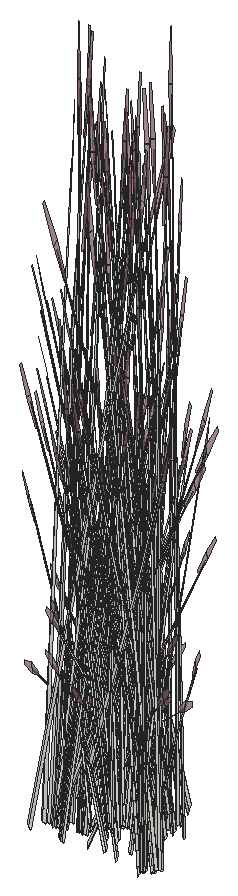
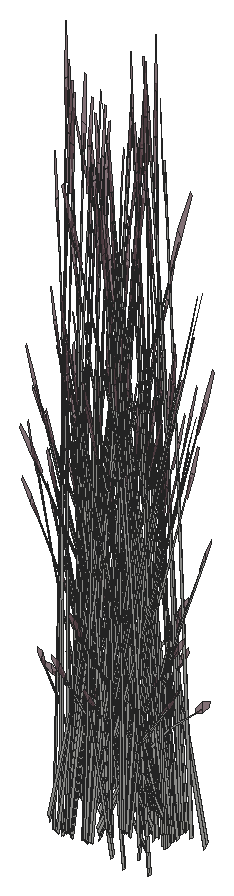
# SketchUp Ruby script. Lengths in inches.
U = 1.inch
M = Sketchup.active_model
def pt(a) = Geom::Point3d.new(a.map { |v| v * U })
def face(e, loops, mat)
  f = e.add_face(loops[0].map { |a| pt(a) })
  loops[1..].each { |l| e.add_face(l.map { |a| pt(a) }).erase! }
  f.material = f.back_material = mat if mat
  f
end
# faces: each face lists its corners as indices into pts; further lists are holes
def faces(e, pts, list, mat = nil) = list.each { |f| face(e, (f[0].is_a?(Array) ? f : [f]).map { |l| l.map { |i| pts[i] } }, mat) }
# xy, xz, yz: faces in a plane at the given z, y or x. An outline is a flat list of corners, or four numbers for a rectangle; further outlines are holes
def ring(l) = l.size == 4 ? [[l[0], l[1]], [l[2], l[1]], [l[2], l[3]], [l[0], l[3]]] : l.each_slice(2).to_a
def flat(e, list, mat, &to3) = list.each { |f| face(e, (f[0].is_a?(Array) ? f : [f]).map { |l| ring(l).map { |u, v| to3.(u, v) } }, mat) }
def xy(e, z, list, mat = nil) = flat(e, list, mat) { |x, y| [x, y, z] }
def xz(e, y, list, mat = nil) = flat(e, list, mat) { |x, z| [x, y, z] }
def yz(e, x, list, mat = nil) = flat(e, list, mat) { |y, z| [x, y, z] }
def lines(e, pts, list) = list.each { |a, b| e.add_line(pt(pts[a]), pt(pts[b])) }
# prism: a flat outline (further loops are holes) pulled along v
def prism(e, loops, v, mat = nil)
  f = face(e, loops, mat); d = Geom::Vector3d.new(v.map { |x| x * U })
  f.pushpull(f.normal.samedirection?(d) ? d.length : -d.length)
end
def box(e, o, s, mat = nil) = prism(e, [[o, [o[0] + s[0], o[1], o[2]], [o[0] + s[0], o[1] + s[1], o[2]], [o[0], o[1] + s[1], o[2]]]], [0, 0, s[2]], mat)
def at(x, y, z, deg = 0) = Geom::Transformation.translation(pt([x, y, z])) * Geom::Transformation.rotation(ORIGIN, Z_AXIS, deg.degrees)
def axes(o, x, y, z) = Geom::Transformation.new([*x, 0, *y, 0, *z, 0, *pt(o).to_a, 1])
def part(name) = M.definitions.add(name)
# library, detail: a bought-in or finely detailed component or shape, given as its bounding box
def library(name, o, s) = part(name).tap { |d| box(d.entities, o, s) }
def detail(e, o, s) = box(e.add_group.entities, o, s)
def put(e, d, t, mat = nil) = e.add_instance(d, t).tap { |i| i.material = mat if mat }
def group(e, t, mat = nil) = e.add_group.tap { |g| g.transformation = t; g.material = mat if mat }.entities
root = M.entities
M.materials.add("LightPink_Translucent").color = [144, 107, 117]
M.materials["LightPink_Translucent"].alpha = 0.75
c1 = part("blade")
p = [[2.15,0.21,22],[0,0.17,0],[0.09,0.45,0],[2.18,0.31,22],[2.29,0.31,22],[0.38,0.45,0],
  [2.48,0.24,33],[2.49,0.24,33],[2.48,0.22,33]]
faces(c1.entities,p,[[0,1,2,3],[4,5,2,3],[6,3,4,7],[8,0,3,6]])
c2 = part("seeds")
p = [[0.3,-0.1,1.38],[-0.01,-0.03,1.59],[-0.01,-0.03,0.03],[0.14,-0.07,-0.07],[0.29,-0.03,3],[0.15,0.01,3.11]]
faces(c2.entities,p,[[0,1,2,3],[1,0,4,5]],"LightPink_Translucent")
c3 = part("blade with seeds")
put(c3.entities,c1,at(0,0,0))
put(c3.entities,c2,axes([2.4,0.25,30.99],[1.5799,-0.05474,1.17369],[-0.12525,1.92788,0.29478],[-0.07173,-0.02425,1.56792]))
put(root,c3,axes([316.8125,31.4,46.4],[0.44368,-0.17257,-0.62776],[0.24726,0.35524,0.07576],[0.21437,-0.04035,0.88802]))
put(root,c3,axes([314.82,30.79,44.09],[-0.41865,0.35461,0.40429],[-0.49737,-0.31303,0.15865],[0.10093,-0.03539,1.40366]))
put(root,c3,axes([321.99,33.24,46],[0.15222,-0.30049,-0.31292],[0.44409,0.08764,0.40398],[-0.04072,-0.12098,0.77298]))
put(root,c3,axes([323.45,30.63,43.9375],[-0.31175,-0.39292,-0.04544],[0.52815,-0.21836,0.456],[-0.13015,0.03741,1.44584]))
put(root,c3,axes([316.75,31.47,46.46],[-0.41962,-0.10901,0.31292],[0.12239,-0.31802,-0.40398],[0.16894,-0.02916,0.77298]))
put(root,c3,axes([323.34,29.68,44.3125],[0.37303,0.23477,0.12794],[-0.31115,0.26487,-0.36534],[-0.08661,0.03581,1.11991]))
put(root,c3,axes([320.4,29.74,46.18],[-0.12522,-0.35963,0.42415],[0.49122,-0.06241,0.34973],[-0.14477,0.08458,0.87768]))
put(root,c3,axes([320.3,29.67,46.18],[-0.34663,-0.16434,0.05682],[0.20181,-0.23402,0.44729],[-0.11113,0.07566,0.68204]))
put(root,c3,axes([321.76,33.44,46.14],[-0.49634,-0.09796,-0.45151],[0.17013,-0.33585,-0.34973],[-0.04551,-0.13522,0.86392]))
put(root,c3,axes([313.875,30.52,43.41],[-0.49699,0.15644,1.13921],[-0.15819,-0.44887,0.44265],[0.30518,0.00747,1.29573]))
put(root,c3,axes([315.21,30.64,44.3125],[0.09741,-0.34873,0.12794],[0.4759,0.06053,-0.36534],[0.08661,0.03581,1.11991]))
put(root,c3,axes([317.76,31.125,43.32],[-0.02639,-0.05932,1.55816],[0.18302,-0.34702,-0.23804],[0.18462,-0.00499,0.26541]))
put(root,c3,axes([320.875,32.4,46.16],[-0.00942,0.04684,1.56736],[-0.46458,0.16998,-0.1481],[-0.13671,-0.08689,0.27737]))
put(root,c3,axes([315.01,30.73,44.4],[-0.30332,-0.32798,0.39531],[0.45944,-0.23096,-0.19025],[0.09816,0.04058,1.26923]))
put(root,c3,axes([323.74,30.4,44.19],[0.47255,-0.19538,0.43871],[0.28245,0.35034,0],[-0.10763,0.0445,1.3917]))
put(root,c3,axes([320.77,33.23,46.5],[0.56246,-0.10044,0.47505],[0.09762,0.39398,0.3917],[-0.13228,-0.11611,0.983]))
put(root,c3,axes([323.3125,30.58,43.79],[-0.47106,-0.09668,-0.27372],[0.11861,-0.34048,0.27372],[-0.09497,0.03926,1.22797]))
put(root,c3,axes([319.91,29.89,44.29],[0.17547,0.03208,1.26356],[0.1131,0.32764,-0.27174],[-0.23835,0.06133,0.54024]))
put(root,c3,axes([315.16,30.75,44.36],[0.50979,-0.25942,-0.25709],[0.339,0.36656,-0.44182],[0.12578,0.03723,1.41118]))
put(root,c3,axes([317.19,31.43,46],[0.41962,0.10901,-0.31292],[-0.12239,0.31802,0.40398],[0.16894,-0.02916,0.77298]))
put(root,c3,axes([322.04,33.31,46.18],[0.49753,0.10215,0.42415],[-0.17013,0.33585,0.34973],[-0.0299,-0.13207,0.87768]))
put(root,c3,axes([322.1875,33.43,46.45],[-0.49409,0.18193,-0.10745],[-0.24281,-0.32289,-0.59638],[-0.06519,-0.13607,0.90619]))
put(root,c3,axes([320.7,29.62,46.46],[0.43951,-0.05584,0.31292],[0.11606,0.31924,-0.40398],[-0.12595,0.08575,0.77298]))
put(root,c3,axes([320.22,32.875,44.44],[0.26338,0.136,1.01491],[-0.38358,0.08175,0.74569],[-0.08207,-0.10452,0.22354]))
put(root,c3,axes([319.01,29.48,46.16],[0.06444,0.01048,1.56736],[0.19934,0.34525,-0.1481],[-0.13191,0.09062,0.27737]))
put(root,c3,axes([322.18,33.28,46.18],[0.37205,-0.1328,0.05682],[0.18211,0.24217,0.44729],[-0.03593,-0.10675,0.68204]))
put(root,c3,axes([320.86,33.6,46.4],[-0.43054,-0.18887,-0.62776],[0.30598,-0.33097,0.07576],[-0.15599,-0.11277,0.88802]))
put(root,c3,axes([316.45,30.06,43.78],[0.47255,0.19538,-0.43871],[-0.28245,0.35034,0],[0.10763,0.0445,1.3917]))
put(root,c3,axes([320.71,33.35,46],[-0.07798,-0.31474,-0.31292],[0.44579,-0.08311,0.40398],[-0.11974,-0.09019,0.77298]))
put(root,c3,axes([315.55,31.17,43.95],[0.56491,0,0],[0,0.40454,0],[0,0,1.5764]))
put(root,c3,axes([319.55,30.57,44.44],[0.21042,-0.1771,1.01491],[0.08303,0.28036,0.74569],[-0.15207,0.0502,0.22354]))
put(root,c3,axes([323.23,29.59,44.36],[0.05884,0.44587,-0.25709],[-0.6128,0.02696,-0.44182],[-0.10791,0.05939,1.41118]))
put(root,c3,axes([320.34,29.81,46],[-0.43951,0.05584,-0.31292],[-0.11606,-0.31924,0.40398],[-0.12595,0.08575,0.77298]))
put(root,c3,axes([316.05,31.04,45.43],[-0.20943,0.00885,1.51428],[0.13893,-0.38357,0.12244],[0.29846,0.02372,0.64734]))
put(root,c3,axes([316.32,30.21,43.79],[0.11861,0.34048,-0.27372],[-0.47106,0.09668,0.27372],[0.09497,0.03926,1.22797]))
put(root,c3,axes([317.13,31.57,46.18],[0.18545,0.26643,0.05682],[-0.33817,0.13041,0.44729],[0.14907,-0.02573,0.68204]))
put(root,c3,axes([320.9,33.32,46.18],[0.22948,-0.24822,0.05682],[0.32679,0.14452,0.44729],[-0.10565,-0.07958,0.68204]))
put(root,c3,axes([320.01,33.28,43.32],[-0.04891,0.05148,1.55816],[-0.49427,0.11098,-0.23804],[-0.1194,-0.10096,0.26541]))
put(root,c3,axes([315.37,30.97,44.1],[-0.63817,-0.08233,0.43472],[0.12987,-0.46497,0.17059],[0.09326,0.0449,1.50931]))
put(root,c3,axes([317.09,31.47,46.18],[-0.14265,0.35629,0.42415],[-0.46898,-0.12183,0.34973],[0.18443,-0.02141,0.87768]))
put(root,c3,axes([319.7,30.53,46.99],[0.44556,0.1043,-0.05733],[-0.13706,0.32103,-0.25992],[-0.07288,0.04874,0.85731]))
put(root,c3,axes([322.86,29.93,43.82],[-0.34009,0.2937,-0.55095],[-0.42248,-0.26632,-0.1446],[-0.13628,0.07327,1.21613]))
put(root,c3,axes([320.83,34.7,43.85],[-0.20736,-0.4007,-0.61707],[0.59731,-0.14431,-0.16195],[-0.02292,-0.13569,1.36206]))
put(root,c3,axes([315.48,32.07,43.93],[0.53009,-0.13258,-0.16963],[0.18627,0.38191,0.00007],[0.05851,-0.01465,1.53656]))
put(root,c3,axes([323.47,30.43,44.06],[0.63212,0.12701,0.27176],[-0.15814,0.45398,-0.32244],[-0.10462,0.05682,1.45692]))
put(root,c3,axes([323.42,30.73,43.78],[-0.47255,0.19538,-0.43871],[-0.28245,-0.35034,0],[-0.10763,0.0445,1.3917]))
put(root,c3,axes([315.54,31.35,43.96],[0.35245,0.2524,0],[-0.35245,0.2524,0],[0,0,1.49564]))
put(root,c3,axes([322.04,33.55,46.46],[-0.15222,0.30049,0.31292],[-0.44409,-0.08764,-0.40398],[-0.04072,-0.12098,0.77298]))
put(root,c3,axes([320.66,33.6,46.14],[-0.49824,0.09289,-0.45151],[-0.08716,-0.35177,-0.34973],[-0.13382,-0.10081,0.86392]))
put(root,c3,axes([315.76,30.81,43.82],[0.52523,0.06406,-0.55095],[-0.11084,0.39517,-0.1446],[0.15674,0.04788,1.21613]))
put(root,c3,axes([318.08,31.5,44.44],[-0.31197,0.06451,1.01491],[0.14684,-0.26661,0.74569],[0.1655,0.01824,0.22354]))
put(root,c3,axes([321,33.29,46.8],[-0.33698,0.3746,-0.12034],[-0.48801,-0.21581,-0.66795],[-0.16964,-0.10584,1.01494]))
put(root,c3,axes([320.47,29.59,46.45],[0.46706,0.21546,-0.10745],[-0.26908,0.31203,-0.59638],[-0.13196,0.10846,0.90619]))
put(root,c3,axes([320.75,33.55,44.1],[-0.31568,-0.39156,0],[0.52815,-0.21836,-0.456],[0.12029,-0.04973,1.44655]))
put(root,c3,axes([315.46,35.08,44.29],[-0.14352,0.07909,1.26356],[-0.42983,-0.13843,-0.27174],[0.07968,-0.17216,0.54024]))
put(root,c3,axes([315.53,31.05,44.4],[0.24498,-0.3521,0.39531],[0.50902,0.16945,-0.19025],[0,0.08116,1.26923]))
put(root,c3,axes([321.1,29.49,45.43],[0.12611,-0.12006,1.51428],[0.31843,0.32408,0.12244],[-0.2184,0.14759,0.64734]))
put(root,c3,axes([317.94,32.625,46.16],[-0.04566,-0.03421,1.56736],[0.09987,-0.36669,-0.1481],[0.17984,-0.02343,0.27737]))
put(root,c3,axes([321.44,33.08,43.88],[-0.34892,0.22417,-0.0344],[-0.3197,-0.24551,-0.15595],[-0.02251,-0.06957,0.51438]))
put(root,c3,axes([320.7,29.85,46.14],[0.12971,0.3568,-0.45151],[-0.49122,0.06241,-0.34973],[-0.14077,0.09583,0.86392]))
put(root,c3,axes([321.29,30.26,46.46],[0.34164,-0.20573,0.31292],[0.3234,0.23491,-0.40398],[-0.04921,0.11936,0.77298]))
put(root,c3,axes([323.85,30.67,44.1],[0.31568,0.39156,0],[-0.52815,0.21836,-0.456],[-0.12029,0.04973,1.44655]))
put(root,c3,axes([315.49,30.93,43.95],[0.30332,0.32798,-0.39531],[-0.45944,0.23096,0.19025],[0.09816,0.04058,1.26923]))
put(root,c3,axes([317.54,32.32,45.47],[-0.09664,-0.32847,-0.03085],[0.45676,-0.07551,-0.13989],[0.09538,0.02082,0.4614]))
put(root,c3,axes([319.71,33.18,46.17],[-0.10864,-0.00276,1.54581],[-0.34587,0.27582,-0.24447],[-0.18454,-0.05636,0.12397]))
put(root,c3,axes([316.35,32.31,46.45],[0.02704,-0.39739,-0.10745],[0.51189,0.01086,-0.59638],[0.19715,0.0276,0.90619]))
put(root,c3,axes([323.58,29.12,44.51],[-0.01379,-0.36791,1.24828],[0.62424,0.09537,0.52853],[-0.14764,0.20132,1.17828]))
put(root,c3,axes([320.98,30.44,46.18],[-0.41493,-0.01821,0.05682],[0.01138,-0.27493,0.44729],[-0.04342,0.10531,0.68204]))
put(root,c3,axes([320.1,30.76,43.32],[0.06773,0.03904,1.55816],[0.11484,0.36171,-0.23804],[-0.15011,0.07713,0.26541]))
put(root,c3,axes([316.82,31.25,44.19],[0,-0.39075,0.43871],[0.56491,0,0],[0,0.089,1.3917]))
put(root,c3,axes([321.12,30.47,46.18],[-0.35954,-0.26661,0.42415],[0.38183,-0.22994,0.34973],[-0.06632,0.12508,0.87768]))
put(root,c3,axes([315.75,31.13,44.3125],[0.47043,-0.11396,0.12794],[0.16474,0.32541,-0.36534],[0,0.07162,1.11991]))
put(root,c3,axes([315.8125,35.67,46.4],[0.01314,-0.36145,-0.62776],[0.55324,0.02428,0.07576],[0.05838,-0.15313,0.88802]))
put(root,c3,axes([321.89,35.73,44.9375],[0.43633,0.15757,1.33654],[-0.42745,0.33945,0.52853],[-0.19146,-0.20119,1.12046]))
put(root,c3,axes([316.28,32.15,46.46],[-0.28729,-0.24465,0.31292],[0.32804,-0.23159,-0.40398],[0.16667,0.03524,0.77298]))
put(root,c3,axes([320.97,33.6,46.46],[0.07798,0.31474,0.31292],[-0.44579,0.08311,-0.40398],[-0.11974,-0.09019,0.77298]))
put(root,c3,axes([319.61,34.64,43.78],[0,-0.39075,-0.43871],[0.56491,0,0],[0,-0.089,1.3917]))
put(root,c3,axes([316.58,35.1,46.17],[-0.00487,-0.07777,1.54581],[-0.41166,-0.22476,-0.24447],[0.06364,-0.13625,0.12397]))
put(root,c3,axes([315.19,35.48,45.43],[-0.09401,0.13431,1.51428],[-0.3944,-0.27795,0.12244],[0.17792,-0.17323,0.64734]))
put(root,c3,axes([316.47,34.82,46.16],[-0.05128,0.02985,1.56736],[-0.5024,-0.1007,-0.1481],[-0.01819,-0.13025,0.27737]))
put(root,c3,axes([319.63,33.81,46.5],[0.41698,-0.28837,0.47505],[0.35962,0.30624,0.3917],[-0.19563,-0.05319,0.983]))
put(root,c3,axes([317.5,31.93,44.29],[-0.1216,-0.0961,1.26356],[0.15822,-0.31792,-0.27174],[0.24603,0.04307,0.54024]))
put(root,c3,axes([315.32,32.27,43.95],[0.50902,0.17543,0],[-0.24498,0.36452,0],[0,0,1.54589]))
put(root,c3,axes([315.7,35.55,46.14],[-0.36145,-0.26255,-0.45151],[0.38183,-0.22994,-0.34973],[0.055,-0.1334,0.86392]))
put(root,c3,axes([316.8,32.07,46.17],[0.10831,-0.00661,1.54581],[0.29709,-0.30358,-0.24447],[0.19266,0.04007,0.12397]))
put(root,c3,axes([321.01,29.79,45.43],[0.09401,-0.13431,1.51428],[0.3944,0.27795,0.12244],[-0.17792,0.17323,0.64734]))
put(root,c3,axes([319.82,33.81,46.18],[0.02542,-0.29714,0.05682],[0.38391,0.00815,0.44729],[-0.14706,-0.03109,0.68204]))
put(root,c3,axes([321.14,34.8,43.95],[0.24498,-0.3521,-0.39531],[0.50902,0.16945,0.19025],[0,-0.08116,1.26923]))
put(root,c3,axes([319.68,33.9,46],[-0.28729,-0.24465,-0.31292],[0.32804,-0.23159,0.40398],[-0.16667,-0.03524,0.77298]))
put(root,c3,axes([319.85,34.65,43.79],[0.35245,-0.2438,-0.27372],[0.35245,0.2438,0.27372],[0,-0.07853,1.22797]))
put(root,c3,axes([322.11,30.87,46.18],[-0.37205,0.1328,0.05682],[-0.18211,-0.24217,0.44729],[0.03593,0.10675,0.68204]))
put(root,c3,axes([321.11,30.55,46],[-0.34164,0.20573,-0.31292],[-0.3234,-0.23491,0.40398],[-0.04921,0.11936,0.77298]))
put(root,c3,axes([319.9375,30.49,46.17],[-0.01255,0.07733,1.54581],[0.35618,0.269,-0.24447],[-0.09325,0.12721,0.12397]))
put(root,c3,axes([316.38,32.12,46.4],[0.50473,0.00941,-0.62776],[-0.0339,0.39618,0.07576],[0.21383,0.04181,0.88802]))
put(root,c3,axes([321.08,30.3125,46.77],[0.55492,0.01936,-0.11927],[-0.01517,0.36657,-0.66198],[-0.03855,0.14118,1.00587]))
put(root,c3,axes([319.71,33.48,43.88],[-0.14565,0.31907,-0.0344],[-0.44829,-0.09815,-0.15595],[-0.06806,-0.05219,0.51438]))
put(root,c3,axes([321.08,35.09,44.36],[-0.56863,-0.18645,-0.25709],[0.2738,-0.39352,-0.44182],[-0.01787,-0.09662,1.41118]))
put(root,c3,axes([322.25,30.84,46.47],[-0.49753,-0.10215,0.47081],[0.17013,-0.33585,0.3882],[0.0299,0.13207,0.97422]))
put(root,c3,axes([316.08,35.68,46.45],[-0.55492,-0.01936,-0.10745],[0.01517,-0.36657,-0.59638],[0.03855,-0.14118,0.90619]))
put(root,c3,axes([316.04,35.45,46],[0.34164,-0.20573,-0.31292],[0.3234,0.23491,0.40398],[0.04921,-0.11936,0.77298]))
put(root,c3,axes([319.47,34.9375,44.1],[-0.63136,0,0],[0,-0.43672,-0.456],[0,-0.09947,1.44655]))
put(root,c3,axes([321.33,31.35,44.44],[-0.01307,-0.23234,1.01491],[0.32652,0.16572,0.74569],[-0.06422,0.11074,0.22354]))
put(root,c3,axes([322.19,30.79,43.32],[0.08172,-0.02126,1.55816],[0.49154,0.11703,-0.23804],[0.01437,0.1319,0.26541]))
put(root,c3,axes([317.2,31.31,44.1],[0.63136,0,0],[0,0.43672,-0.456],[0,0.09947,1.44655]))
put(root,c3,axes([315.59,31.16,44.36],[0.56863,0.18645,-0.25709],[-0.2738,0.39352,-0.44182],[0.01787,0.09662,1.41118]))
put(root,c3,axes([321.45,30.45,46.42],[0.36145,0.26255,-0.50118],[-0.38183,0.22994,-0.3882],[-0.055,0.1334,0.95895]))
put(root,c3,axes([316.68,32.28,46],[0.28729,0.24465,-0.31292],[-0.32804,0.23159,0.40398],[0.16667,0.03524,0.77298]))
put(root,c3,axes([316.82,31.6,43.79],[-0.35245,0.2438,-0.27372],[-0.35245,-0.2438,0.27372],[0,0.07853,1.22797]))
put(root,c3,axes([321.0625,30.84,44.49],[0.45869,-0.0692,0.0575],[0.10545,0.27878,-0.76259],[-0.02908,0.14112,0.68355]))
put(root,c3,axes([316.54,32.375,46.18],[-0.02542,0.29714,0.05682],[-0.38391,-0.00815,0.44729],[0.14706,0.03109,0.68204]))
put(root,c3,axes([316.57,32.28,46.18],[-0.3723,0.25748,0.42415],[-0.32109,-0.27343,0.34973],[0.17467,0.04749,0.87768]))
put(root,c3,axes([322.3,30.91,46],[-0.15222,0.30049,-0.31292],[-0.44409,-0.08764,0.40398],[0.04072,0.12098,0.77298]))
put(root,c3,axes([316.47,35.32,43.32],[-0.07557,-0.03078,1.55816],[-0.19412,-0.34391,-0.23804],[0.13095,-0.09333,0.26541]))
put(root,c3,axes([319.95,34.82,44.06],[-0.46965,0.32852,0.27176],[-0.46994,-0.32506,-0.32244],[-0.0164,-0.09329,1.45692]))
put(root,c3,axes([319.3,33.42,46.16],[0.03743,0.039,1.56736],[-0.18045,0.35054,-0.1481],[-0.18276,0.00254,0.27737]))
put(root,c3,axes([321.34,30.33,46.72],[-0.01314,0.36145,-0.69681],[-0.55324,-0.02428,0.08409],[-0.05838,0.15313,0.9857]))
put(root,c3,axes([319.9,31.28,46.16],[0.05728,-0.02359,1.56736],[0.47345,0.15692,-0.1481],[-0.01113,0.13066,0.27737]))
put(root,c3,axes([321.45,34.98,44.15],[0.56891,0.18939,0.21263],[-0.2738,0.39352,0.44182],[0,-0.09071,1.41855]))
put(root,c3,axes([316.04,35.53,46.18],[0.35954,0.26661,0.42415],[-0.38183,0.22994,0.34973],[0.06632,-0.12508,0.87768]))
put(root,c3,axes([321.23,35.51,44.16],[0.13383,-0.46302,-0.20702],[0.63453,0.08071,0.45303],[-0.11087,-0.06394,1.38231]))
put(root,c3,axes([316.17,35.55,46.18],[0.41493,0.01821,0.05682],[-0.01138,0.27493,0.44729],[0.04342,-0.10531,0.68204]))
put(root,c3,axes([315.39,32.58,46.46],[-0.07798,-0.31474,0.31292],[0.44579,-0.08311,-0.40398],[0.11974,0.09019,0.77298]))
put(root,c3,axes([319.8125,34.14,46.14],[-0.36663,0.25884,-0.45151],[-0.32109,-0.27343,-0.34973],[-0.18628,-0.03938,0.86392]))
put(root,c3,axes([321.87,30.07,45.43],[-0.01236,-0.14998,1.51428],[0.53562,0.09949,0.12244],[-0.03313,0.21373,0.64734]))
put(root,c3,axes([317.0625,31.61,43.78],[0,0.39075,-0.43871],[-0.56491,0,0],[0,0.089,1.3917]))
put(root,c3,axes([320.08,34.03,46.46],[0.28729,0.24465,0.31292],[-0.32804,0.23159,-0.40398],[-0.16667,-0.03524,0.77298]))
put(root,c3,axes([315.65,31.65,45.43],[-0.18755,-0.06732,1.51428],[0.38813,-0.28243,0.12244],[0.24191,0.12741,0.64734]))
put(root,c3,axes([318.99,34.49,44.44],[0.32236,-0.02796,1.01491],[-0.20448,0.24636,0.74569],[-0.1593,-0.03696,0.22354]))
put(root,c3,axes([315.86,35.74,46.46],[-0.34164,0.20573,0.31292],[-0.3234,-0.23491,-0.40398],[0.04921,-0.11936,0.77298]))
put(root,c3,axes([315.6875,30.77,45.95],[-0.4363,-0.20303,1.22187],[0.46069,-0.31611,0.5272],[0.14077,0.1905,1.18105]))
put(root,c3,axes([316.46,36.29,46.4],[0.26374,-0.30832,-0.62776],[0.46217,0.21911,0.07576],[0.15748,-0.11171,0.88802]))
put(root,c3,axes([316.45,36.15,46.14],[-0.12971,-0.3568,-0.45151],[0.49122,-0.06241,-0.34973],[0.14077,-0.09583,0.86392]))
put(root,c3,axes([321.26,34.71,44.4],[-0.54829,0.02412,0.39531],[-0.04958,-0.40041,-0.19025],[0.09816,-0.04058,1.26923]))
put(root,c3,axes([320.01,33.87,46.45],[-0.02704,0.39739,-0.10745],[-0.51189,-0.01086,-0.59638],[-0.19715,-0.0276,0.90619]))
put(root,c3,axes([319.85,35.01,44.19],[0,0.39075,0.43871],[-0.56491,0,0],[0,-0.089,1.3917]))
put(root,c3,axes([316.35,32.42,44.44],[-0.28429,-0.11236,1.01491],[0.36709,-0.11416,0.74569],[0.09901,0.0967,0.22354]))
put(root,c3,axes([320.95,31.14,44.29],[0.15933,-0.06164,1.26356],[0.39339,0.18587,-0.27174],[-0.11709,0.16083,0.54024]))
put(root,c3,axes([315.35,32.74,46.45],[0.30087,-0.33447,-0.10745],[0.43572,0.19269,-0.59638],[0.15146,0.0945,0.90619]))
put(root,c3,axes([321.18,35.32,43.95],[-0.30332,-0.32798,-0.39531],[0.45944,-0.23096,0.19025],[-0.09816,-0.04058,1.26923]))
put(root,c3,axes([321.25,34.86,44.09],[0.21952,0.43694,0.40429],[-0.62724,0.15194,0.15865],[0.00767,-0.08029,1.40366]))
put(root,c3,axes([316.68,36.41,46.45],[-0.46706,-0.21546,-0.10745],[0.26908,-0.31203,-0.59638],[0.13196,-0.10846,0.90619]))
put(root,c3,axes([321.14,35.2,44.4],[-0.24498,0.3521,0.39531],[-0.50902,-0.16945,-0.19025],[0,-0.08116,1.26923]))
put(root,c3,axes([322.03,34.89,43.95],[0,-0.45213,0],[0.63136,0,0],[0,0,1.58567]))
put(root,c3,axes([314.95,33.02,46.16],[0.00149,-0.04731,1.56736],[0.4327,-0.20872,-0.1481],[0.1503,0.0745,0.27737]))
put(root,c3,axes([316.42,32.84,43.32],[0.03679,-0.05641,1.55816],[0.46313,-0.16615,-0.23804],[0.14041,0.08599,0.26541]))
put(root,c3,axes([315.8125,31.56,43.85],[0.18514,0.35777,-0.61156],[-0.53331,0.12885,-0.16051],[0.02046,0.12115,1.3499]))
put(root,c3,axes([314.04,35.34,43.78],[0.47255,-0.19538,-0.43871],[0.28245,0.35034,0],[0.10763,-0.0445,1.3917]))
put(root,c3,axes([316.85,36.01,44.29],[-0.18038,-0.01157,1.26356],[-0.18479,-0.31048,-0.27174],[0.22159,-0.08783,0.54024]))
